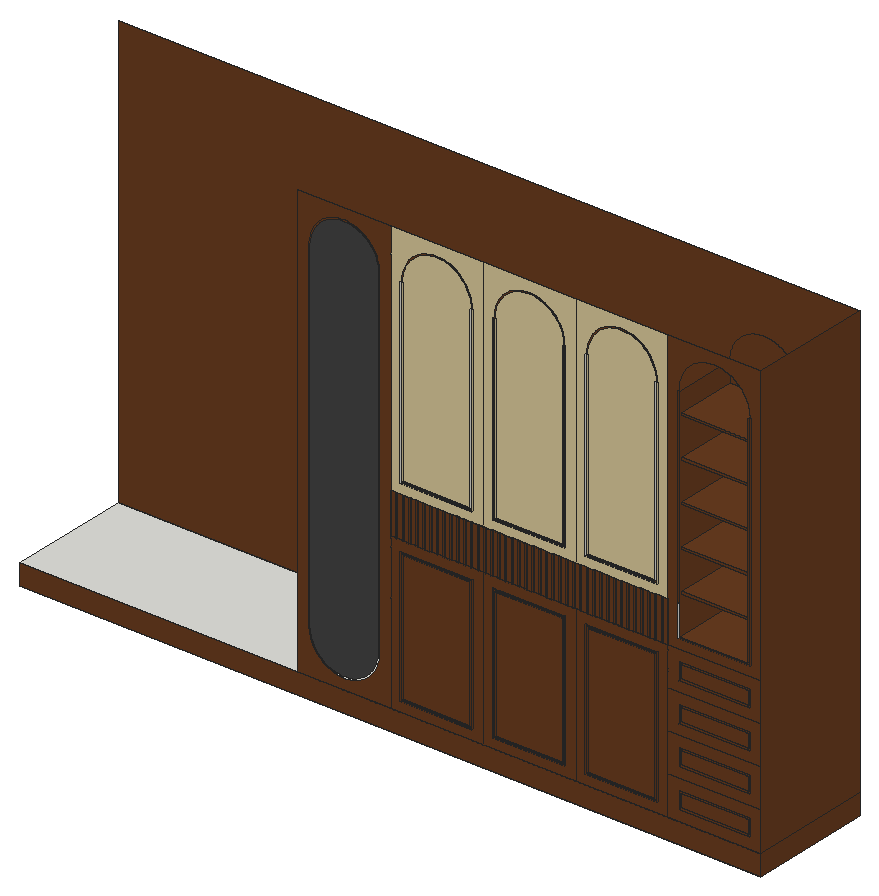
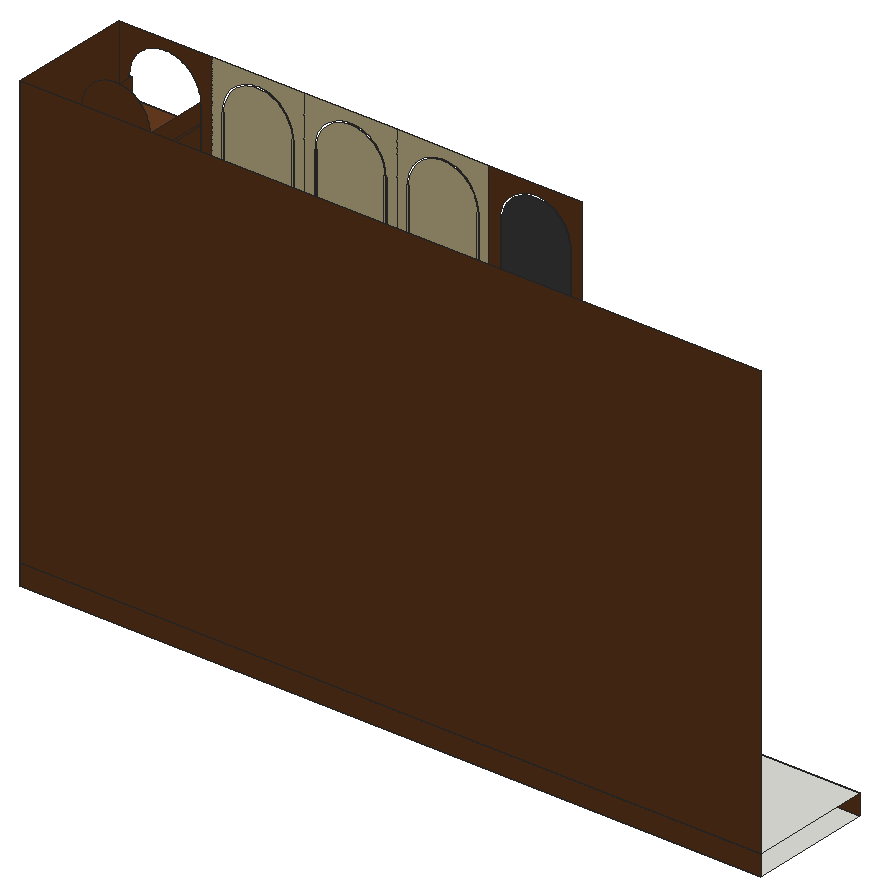
# SketchUp Ruby script. Lengths in inches.
U = 1.inch
M = Sketchup.active_model
def pt(a) = Geom::Point3d.new(a.map { |v| v * U })
def face(e, loops, mat)
  f = e.add_face(loops[0].map { |a| pt(a) })
  loops[1..].each { |l| e.add_face(l.map { |a| pt(a) }).erase! }
  f.material = f.back_material = mat if mat
  f
end
# faces: each face lists its corners as indices into pts; further lists are holes
def faces(e, pts, list, mat = nil) = list.each { |f| face(e, (f[0].is_a?(Array) ? f : [f]).map { |l| l.map { |i| pts[i] } }, mat) }
# xy, xz, yz: faces in a plane at the given z, y or x. An outline is a flat list of corners, or four numbers for a rectangle; further outlines are holes
def ring(l) = l.size == 4 ? [[l[0], l[1]], [l[2], l[1]], [l[2], l[3]], [l[0], l[3]]] : l.each_slice(2).to_a
def flat(e, list, mat, &to3) = list.each { |f| face(e, (f[0].is_a?(Array) ? f : [f]).map { |l| ring(l).map { |u, v| to3.(u, v) } }, mat) }
def xy(e, z, list, mat = nil) = flat(e, list, mat) { |x, y| [x, y, z] }
def xz(e, y, list, mat = nil) = flat(e, list, mat) { |x, z| [x, y, z] }
def yz(e, x, list, mat = nil) = flat(e, list, mat) { |y, z| [x, y, z] }
def lines(e, pts, list) = list.each { |a, b| e.add_line(pt(pts[a]), pt(pts[b])) }
# prism: a flat outline (further loops are holes) pulled along v
def prism(e, loops, v, mat = nil)
  f = face(e, loops, mat); d = Geom::Vector3d.new(v.map { |x| x * U })
  f.pushpull(f.normal.samedirection?(d) ? d.length : -d.length)
end
def box(e, o, s, mat = nil) = prism(e, [[o, [o[0] + s[0], o[1], o[2]], [o[0] + s[0], o[1] + s[1], o[2]], [o[0], o[1] + s[1], o[2]]]], [0, 0, s[2]], mat)
def at(x, y, z, deg = 0) = Geom::Transformation.translation(pt([x, y, z])) * Geom::Transformation.rotation(ORIGIN, Z_AXIS, deg.degrees)
def axes(o, x, y, z) = Geom::Transformation.new([*x, 0, *y, 0, *z, 0, *pt(o).to_a, 1])
def part(name) = M.definitions.add(name)
# library, detail: a bought-in or finely detailed component or shape, given as its bounding box
def library(name, o, s) = part(name).tap { |d| box(d.entities, o, s) }
def detail(e, o, s) = box(e.add_group.entities, o, s)
def put(e, d, t, mat = nil) = e.add_instance(d, t).tap { |i| i.material = mat if mat }
def group(e, t, mat = nil) = e.add_group.tap { |g| g.transformation = t; g.material = mat if mat }.entities
root = M.entities
M.materials.add("138_plaster painted wall texture-seamless").color = [214, 198, 153]
M.materials.add("[Translucent Glass Gray]").color = [66, 66, 66]
M.materials.add("[Wood Veneer 01]").color = [104, 60, 32]
c1 = part("Square post")
box(c1.entities,[0,0,0],[1,1,8])
c2 = part("Group\#15")
box(c2.entities,[0,0,0],[13.2,12,0.4])
xy(root,0,[[24,120,168,144]])
xy(root,4,[[24,120,168,144]])
xy(root,6,[[98,119.8,112,120],[116,119.8,130,120],[134,119.8,148,120]],"[Wood Veneer 01]")
xy(root,6.4,[[98.4,119.8,111.6,120],[116.4,119.8,129.6,120],[134.4,119.8,147.6,120],[152.4,120,165.6,120.2]],"[Wood Veneer 01]")
xy(root,9.1,[[152.4,120,165.6,120.2]])
xy(root,13.9,[[152.4,120,165.6,120.2]],"[Wood Veneer 01]")
xy(root,16.6,[[152.4,120,165.6,120.2]])
xy(root,21.4,[[152.4,120,165.6,120.2]],"[Wood Veneer 01]")
xy(root,24.1,[[152.4,120,165.6,120.2]])
xy(root,28.9,[[152.4,120,165.6,120.2]],"[Wood Veneer 01]")
xy(root,31.6,[[98.4,119.8,111.6,120],[116.4,119.8,129.6,120],[152.4,120,165.6,120.2]])
xy(root,31.6,[[134.4,119.8,147.6,120]],"[Wood Veneer 01]")
xy(root,32,[[98,119.8,112,120],[116,119.8,130,120],[134,119.8,148,120]],"[Wood Veneer 01]")
xy(root,34,[[96,120,114,121],[114,120,132,121],[132,120,150,121]])
xy(root,36,[[152,119.8,166,120]],"[Wood Veneer 01]")
xy(root,36.4,[[152.4,119.8,165.6,132]],"[Wood Veneer 01]")
xy(root,42,[[96,120,114,121],[114,120,132,121],[132,120,150,121]])
xy(root,44,[[98,119.8,112,120],[116,119.8,130,120],[134,119.8,148,120]])
xy(root,44.4,[[98.4,119.8,111.6,120],[116.4,119.8,129.6,120],[134.4,119.8,147.6,120]])
xz(root,120,[[[96,42,114,88],[98,44,98,79,98.01,79.46,98.06,79.91,98.13,80.37,98.24,80.8125,98.37,81.25,98.53,81.68,98.72,82.1,98.9375,82.5,99.18,82.89,99.45,83.26,99.74,83.62,100.05,83.95,100.38,84.26,100.74,84.55,101.11,84.82,101.5,85.0625,101.9,85.28,102.32,85.47,102.75,85.63,103.1875,85.76,103.63,85.87,104.09,85.94,104.54,85.99,105,86,105.46,85.99,105.91,85.94,106.37,85.87,106.8125,85.76,107.25,85.63,107.68,85.47,108.1,85.28,108.5,85.0625,108.89,84.82,109.26,84.55,109.62,84.26,109.95,83.95,110.26,83.62,110.55,83.26,110.82,82.89,111.0625,82.5,111.28,82.1,111.47,81.68,111.63,81.25,111.76,80.8125,111.87,80.37,111.94,79.91,111.99,79.46,112,79,112,44]],[[114,42,132,88],[116,44,116,79,116.01,79.46,116.06,79.91,116.13,80.37,116.24,80.8125,116.37,81.25,116.53,81.68,116.72,82.1,116.9375,82.5,117.18,82.89,117.45,83.26,117.74,83.62,118.05,83.95,118.38,84.26,118.74,84.55,119.11,84.82,119.5,85.0625,119.9,85.28,120.32,85.47,120.75,85.63,121.1875,85.76,121.63,85.87,122.09,85.94,122.54,85.99,123,86,123.46,85.99,123.91,85.94,124.37,85.87,124.8125,85.76,125.25,85.63,125.68,85.47,126.1,85.28,126.5,85.0625,126.89,84.82,127.26,84.55,127.62,84.26,127.95,83.95,128.26,83.62,128.55,83.26,128.82,82.89,129.0625,82.5,129.28,82.1,129.47,81.68,129.63,81.25,129.76,80.8125,129.87,80.37,129.94,79.91,129.99,79.46,130,79,130,44]],[[132,42,150,88],[134,44,134,79,134.01,79.46,134.06,79.91,134.13,80.37,134.24,80.8125,134.37,81.25,134.53,81.68,134.72,82.1,134.9375,82.5,135.18,82.89,135.45,83.26,135.74,83.62,136.05,83.95,136.38,84.26,136.74,84.55,137.11,84.82,137.5,85.0625,137.9,85.28,138.32,85.47,138.75,85.63,139.1875,85.76,139.63,85.87,140.09,85.94,140.54,85.99,141,86,141.46,85.99,141.91,85.94,142.37,85.87,142.8125,85.76,143.25,85.63,143.68,85.47,144.1,85.28,144.5,85.0625,144.89,84.82,145.26,84.55,145.62,84.26,145.95,83.95,146.26,83.62,146.55,83.26,146.82,82.89,147.0625,82.5,147.28,82.1,147.47,81.68,147.63,81.25,147.76,80.8125,147.87,80.37,147.94,79.91,147.99,79.46,148,79,148,44]],[98.4,44.4,111.6,44.4,111.6,79,111.59,79.43,111.54,79.86,111.47,80.29,111.375,80.71,111.25,81.12,111.1,81.53,110.92,81.92,110.72,82.3,110.49,82.67,110.24,83.02,109.96,83.35,109.67,83.67,109.35,83.96,109.02,84.24,108.67,84.49,108.3,84.72,107.92,84.92,107.53,85.1,107.12,85.25,106.71,85.375,106.29,85.47,105.86,85.54,105.43,85.59,105,85.6,104.57,85.59,104.14,85.54,103.71,85.47,103.29,85.375,102.88,85.25,102.47,85.1,102.08,84.92,101.7,84.72,101.33,84.49,100.98,84.24,100.65,83.96,100.33,83.67,100.04,83.35,99.76,83.02,99.51,82.67,99.28,82.3,99.08,81.92,98.9,81.53,98.75,81.12,98.625,80.71,98.53,80.29,98.46,79.86,98.41,79.43,98.4,79],[116.4,44.4,129.6,44.4,129.6,79,129.59,79.43,129.54,79.86,129.47,80.29,129.375,80.71,129.25,81.12,129.1,81.53,128.92,81.92,128.72,82.3,128.49,82.67,128.24,83.02,127.96,83.35,127.67,83.67,127.35,83.96,127.02,84.24,126.67,84.49,126.3,84.72,125.92,84.92,125.53,85.1,125.12,85.25,124.71,85.375,124.29,85.47,123.86,85.54,123.43,85.59,123,85.6,122.57,85.59,122.14,85.54,121.71,85.47,121.29,85.375,120.88,85.25,120.47,85.1,120.08,84.92,119.7,84.72,119.33,84.49,118.98,84.24,118.65,83.96,118.33,83.67,118.04,83.35,117.76,83.02,117.51,82.67,117.28,82.3,117.08,81.92,116.9,81.53,116.75,81.12,116.625,80.71,116.53,80.29,116.46,79.86,116.41,79.43,116.4,79],
  [134.4,44.4,147.6,44.4,147.6,79,147.59,79.43,147.54,79.86,147.47,80.29,147.375,80.71,147.25,81.12,147.1,81.53,146.92,81.92,146.72,82.3,146.49,82.67,146.24,83.02,145.96,83.35,145.67,83.67,145.35,83.96,145.02,84.24,144.67,84.49,144.3,84.72,143.92,84.92,143.53,85.1,143.12,85.25,142.71,85.375,142.29,85.47,141.86,85.54,141.43,85.59,141,85.6,140.57,85.59,140.14,85.54,139.71,85.47,139.29,85.375,138.88,85.25,138.47,85.1,138.08,84.92,137.7,84.72,137.33,84.49,136.98,84.24,136.65,83.96,136.33,83.67,136.04,83.35,135.76,83.02,135.51,82.67,135.28,82.3,135.08,81.92,134.9,81.53,134.75,81.12,134.625,80.71,134.53,80.29,134.46,79.86,134.41,79.43,134.4,79]],"138_plaster painted wall texture-seamless")
xz(root,120,[[87,6.4,87.43,6.41,87.86,6.46,88.29,6.53,88.71,6.625,89.12,6.75,89.53,6.9,89.92,7.08,90.3,7.28,90.67,7.51,91.02,7.76,91.35,8.04,91.67,8.33,91.96,8.65,92.24,8.98,92.49,9.33,92.72,9.7,92.92,10.08,93.1,10.47,93.25,10.88,93.375,11.29,93.47,11.71,93.54,12.14,93.59,12.57,93.6,13,93.6,79,93.59,79.43,93.54,79.86,93.47,80.29,93.375,80.71,93.25,81.12,93.1,81.53,92.92,81.92,92.72,82.3,92.49,82.67,92.24,83.02,91.96,83.35,91.67,83.67,91.35,83.96,91.02,84.24,90.67,84.49,90.3,84.72,89.92,84.92,89.53,85.1,89.12,85.25,88.71,85.375,88.29,85.47,87.86,85.54,87.43,85.59,87,85.6,86.57,85.59,86.14,85.54,85.71,85.47,85.29,85.375,84.88,85.25,84.47,85.1,84.08,84.92,83.7,84.72,83.33,84.49,82.98,84.24,82.65,83.96,82.33,83.67,82.04,83.35,81.76,83.02,81.51,82.67,81.28,82.3,81.08,81.92,80.9,81.53,80.75,81.12,80.625,80.71,80.53,80.29,80.46,79.86,80.41,79.43,80.4,79,80.4,13,80.41,12.57,80.46,12.14,80.53,11.71,80.625,11.29,80.75,10.88,80.9,10.47,81.08,10.08,81.28,9.7,81.51,9.33,81.76,8.98,82.04,8.65,82.33,8.33,82.65,8.04,82.98,7.76,83.33,7.51,83.7,7.28,84.08,7.08,84.47,6.9,84.88,6.75,85.29,6.625,85.71,6.53,86.14,6.46,86.57,6.41]],"[Translucent Glass Gray]")
xz(root,120,[[24,0,168,4],[[78,4,96,88],[87,6,86.54,6.01,86.09,6.06,85.63,6.13,85.1875,6.24,84.75,6.37,84.32,6.53,83.9,6.72,83.5,6.9375,83.11,7.18,82.74,7.45,82.38,7.74,82.05,8.05,81.74,8.38,81.45,8.74,81.18,9.11,80.9375,9.5,80.72,9.9,80.53,10.32,80.37,10.75,80.24,11.1875,80.13,11.63,80.06,12.09,80.01,12.54,80,13,80,79,80.01,79.46,80.06,79.91,80.13,80.37,80.24,80.8125,80.37,81.25,80.53,81.68,80.72,82.1,80.9375,82.5,81.18,82.89,81.45,83.26,81.74,83.62,82.05,83.95,82.38,84.26,82.74,84.55,83.11,84.82,83.5,85.0625,83.9,85.28,84.32,85.47,84.75,85.63,85.1875,85.76,85.63,85.87,86.09,85.94,86.54,85.99,87,86,87.46,85.99,87.91,85.94,88.37,85.87,88.8125,85.76,89.25,85.63,89.68,85.47,90.1,85.28,90.5,85.0625,90.89,84.82,91.26,84.55,91.62,84.26,91.95,83.95,92.26,83.62,92.55,83.26,92.82,82.89,93.0625,82.5,93.28,82.1,93.47,81.68,93.63,81.25,93.76,80.8125,93.87,80.37,93.94,79.91,93.99,79.46,94,79,94,13,93.99,12.54,93.94,12.09,93.87,11.63,93.76,11.1875,93.63,10.75,93.47,10.32,93.28,9.9,93.0625,9.5,92.82,9.11,92.55,8.74,92.26,8.38,91.95,8.05,91.62,7.74,91.26,7.45,90.89,7.18,90.5,6.9375,90.1,6.72,89.68,6.53,89.25,6.37,88.8125,6.24,88.37,6.13,87.91,6.06,87.46,6.01]],[[96,4,114,34],[98,6,112,32]],[[114,4,132,34],[116,6,130,32]],[[132,4,150,34],[134,6,148,32]],
  [[150,4,168,11.5],[152,6,166,9.5]],[[152,6,166,9.5],[152.4,6.4,165.6,9.1]],[98.4,6.4,111.6,31.6],[116.4,6.4,129.6,31.6],[134.4,6.4,147.6,31.6],
  [[150,11.5,168,19],[152,13.5,166,17]],[[152,13.5,166,17],[152.4,13.9,165.6,16.6]],[[150,19,168,26.5],[152,21,166,24.5]],[[152,21,166,24.5],[152.4,21.4,165.6,24.1]],[[150,26.5,168,34],[152,28.5,166,32]],
  [[152,28.5,166,32],[152.4,28.9,165.6,31.6]],[[150,34,168,88],[152,36,152,79,152.01,79.39,152.04,79.77,152.1,80.15,152.17,80.53,152.26,80.9,152.38,81.27,152.51,81.63,152.67,81.99,152.84,82.33,153.04,82.67,153.25,82.99,153.48,83.3,153.72,83.6,153.98,83.88,154.26,84.15,154.55,84.4,154.85,84.64,155.17,84.86,155.5,85.0625,155.84,85.25,156.1875,85.41,156.55,85.56,156.91,85.68,157.28,85.79,157.66,85.87,158.04,85.93,158.42,85.98,158.81,86,159.19,86,159.58,85.98,159.96,85.93,160.34,85.87,160.72,85.79,161.09,85.68,161.45,85.56,161.8125,85.41,162.16,85.25,162.5,85.0625,162.83,84.86,163.15,84.64,163.45,84.4,163.74,84.15,164.02,83.88,164.28,83.6,164.52,83.3,164.75,82.99,164.96,82.67,165.16,82.33,165.33,81.99,165.49,81.63,165.62,81.27,165.74,80.9,165.83,80.53,165.9,80.15,165.96,79.77,165.99,79.39,166,79,166,36]]],"[Wood Veneer 01]")
xz(root,120.2,[[152.4,6.4,165.6,9.1],[152.4,13.9,165.6,16.6],[152.4,21.4,165.6,24.1],[152.4,28.9,165.6,31.6]],"[Wood Veneer 01]")
xz(root,121,[[96,34,150,42]],"[Wood Veneer 01]")
xz(root,132,[[152.4,36.4,165.6,36.4,165.6,79,165.59,79.36,165.56,79.73,165.51,80.09,165.44,80.44,165.35,80.8,165.24,81.14,165.11,81.48,164.97,81.82,164.8,82.14,164.62,82.46,164.42,82.76,164.21,83.05,163.98,83.33,163.73,83.6,163.47,83.86,163.2,84.09,162.91,84.32,162.61,84.53,162.3,84.72,161.98,84.89,161.65,85.04,161.3125,85.18,160.97,85.3,160.62,85.4,160.27,85.48,159.91,85.54,159.55,85.58,159.18,85.6,158.82,85.6,158.45,85.58,158.09,85.54,157.73,85.48,157.38,85.4,157.03,85.3,156.6875,85.18,156.35,85.04,156.02,84.89,155.7,84.72,155.39,84.53,155.09,84.32,154.8,84.09,154.53,83.86,154.27,83.6,154.02,83.33,153.79,83.05,153.58,82.76,153.38,82.46,153.2,82.14,153.03,81.82,152.89,81.48,152.76,81.14,152.65,80.8,152.56,80.44,152.49,80.09,152.44,79.73,152.41,79.36,152.4,79]],"[Wood Veneer 01]")
xz(root,144,[[24,0,168,4],[24,4,168,88]],"[Wood Veneer 01]")
yz(root,96,[[120,34,121,42]])
yz(root,98,[[119.8,44,120,79]])
yz(root,98,[[119.8,6,120,32]],"[Wood Veneer 01]")
yz(root,98.4,[[119.8,44.4,120,79]],"138_plaster painted wall texture-seamless")
yz(root,98.4,[[119.8,6.4,120,31.6]],"[Wood Veneer 01]")
yz(root,111.6,[[119.8,44.4,120,79]])
yz(root,111.6,[[119.8,6.4,120,31.6]],"[Wood Veneer 01]")
yz(root,112,[[119.8,44,120,79]],"138_plaster painted wall texture-seamless")
yz(root,112,[[119.8,6,120,32]],"[Wood Veneer 01]")
yz(root,116,[[119.8,44,120,79]])
yz(root,116,[[119.8,6,120,32]],"[Wood Veneer 01]")
yz(root,116.4,[[119.8,44.4,120,79]],"138_plaster painted wall texture-seamless")
yz(root,116.4,[[119.8,6.4,120,31.6]],"[Wood Veneer 01]")
yz(root,129.6,[[119.8,44.4,120,79]])
yz(root,129.6,[[119.8,6.4,120,31.6]],"[Wood Veneer 01]")
yz(root,130,[[119.8,44,120,79]],"138_plaster painted wall texture-seamless")
yz(root,130,[[119.8,6,120,32]],"[Wood Veneer 01]")
yz(root,134,[[119.8,44,120,79]])
yz(root,134,[[119.8,6,120,32]],"[Wood Veneer 01]")
yz(root,134.4,[[119.8,44.4,120,79]],"138_plaster painted wall texture-seamless")
yz(root,134.4,[[119.8,6.4,120,31.6]],"[Wood Veneer 01]")
yz(root,147.6,[[119.8,44.4,120,79]])
yz(root,147.6,[[119.8,6.4,120,31.6]],"[Wood Veneer 01]")
yz(root,148,[[119.8,44,120,79]],"138_plaster painted wall texture-seamless")
yz(root,148,[[119.8,6,120,32]],"[Wood Veneer 01]")
yz(root,150,[[120,34,121,42]])
yz(root,152,[[119.8,36,120,42]])
yz(root,152,[[119.8,42,120,79]],"[Wood Veneer 01]")
yz(root,152.4,[[120,6.4,120.2,9.1],[120,13.9,120.2,16.6],[120,21.4,120.2,24.1],[120,28.9,120.2,31.6],[119.8,36.4,132,79]],"[Wood Veneer 01]")
yz(root,165.6,[[120,6.4,120.2,9.1],[120,13.9,120.2,16.6],[120,21.4,120.2,24.1],[120,28.9,120.2,31.6],[119.8,36.4,132,79]],"[Wood Veneer 01]")
yz(root,166,[[119.8,36,120,79]],"[Wood Veneer 01]")
yz(root,168,[[120,0,144,4],[120,4,144,88]],"[Wood Veneer 01]")
g1 = group(root,at(96,120,34),"[Wood Veneer 01]")
put(g1,c1,at(6.625,0,0))
put(g1,c1,at(27.82,0,0))
put(g1,c1,at(1.33,0,0))
put(g1,c1,at(3.97,0,0))
put(g1,c1,at(2.65,0,0))
put(g1,c1,at(5.3,0,0))
put(g1,c1,at(0,0,0))
put(g1,c1,at(46.375,0,0))
put(g1,c1,at(47.7,0,0))
put(g1,c1,at(33.125,0,0))
put(g1,c1,at(39.75,0,0))
put(g1,c1,at(31.8,0,0))
put(g1,c1,at(35.78,0,0))
put(g1,c1,at(34.45,0,0))
put(g1,c1,at(43.73,0,0))
put(g1,c1,at(45.05,0,0))
put(g1,c1,at(38.43,0,0))
put(g1,c1,at(30.47,0,0))
put(g1,c1,at(42.4,0,0))
put(g1,c1,at(29.15,0,0))
put(g1,c1,at(41.08,0,0))
put(g1,c1,at(37.1,0,0))
put(g1,c1,at(14.58,0,0))
put(g1,c1,at(7.95,0,0))
put(g1,c1,at(18.55,0,0))
put(g1,c1,at(19.875,0,0))
put(g1,c1,at(25.17,0,0))
put(g1,c1,at(26.5,0,0))
put(g1,c1,at(11.92,0,0))
put(g1,c1,at(13.25,0,0))
put(g1,c1,at(22.52,0,0))
put(g1,c1,at(17.22,0,0))
put(g1,c1,at(10.6,0,0))
put(g1,c1,at(49.03,0,0))
put(g1,c1,at(9.28,0,0))
put(g1,c1,at(21.2,0,0))
put(g1,c1,at(23.85,0,0))
put(g1,c1,at(15.9,0,0))
put(g1,c1,at(50.35,0,0))
put(g1,c1,at(51.68,0,0))
put(g1,c1,at(53,0,0))
g2 = group(root,at(152.4,120,43.78),"[Wood Veneer 01]")
put(g2,c2,at(0,0,7.77))
put(g2,c2,at(0,0,31.1))
put(g2,c2,at(0,0,0))
put(g2,c2,at(0,0,15.55))
put(g2,c2,at(0,0,23.33))
